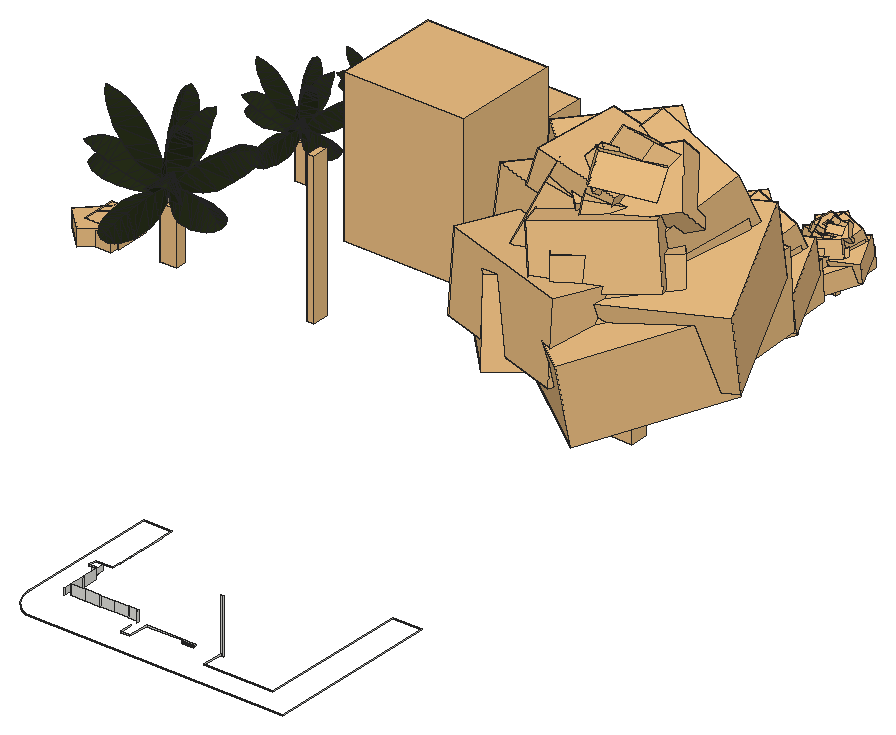
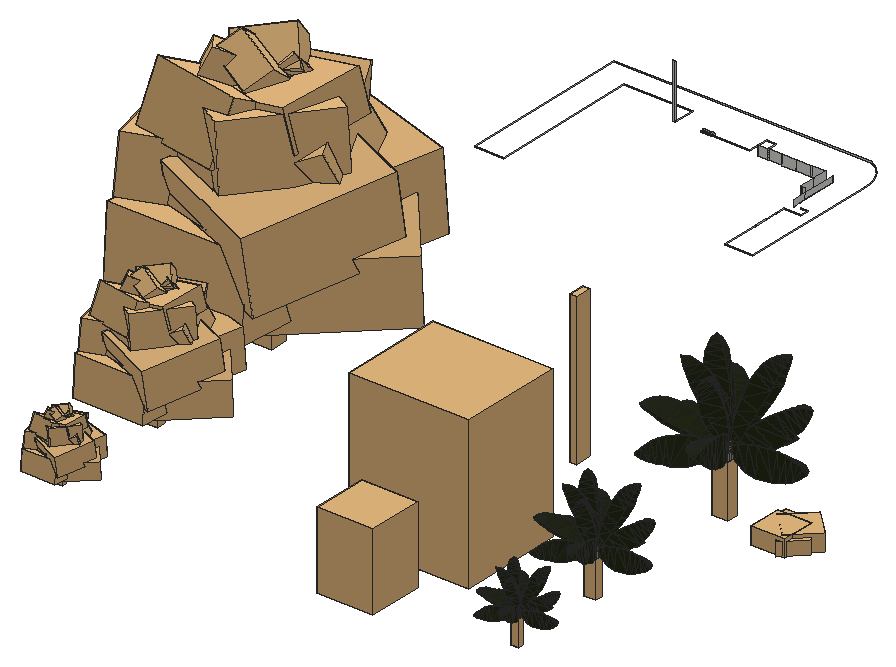
# SketchUp Ruby script. Lengths in inches.
U = 1.inch
M = Sketchup.active_model
def pt(a) = Geom::Point3d.new(a.map { |v| v * U })
def face(e, loops, mat)
  f = e.add_face(loops[0].map { |a| pt(a) })
  loops[1..].each { |l| e.add_face(l.map { |a| pt(a) }).erase! }
  f.material = f.back_material = mat if mat
  f
end
# faces: each face lists its corners as indices into pts; further lists are holes
def faces(e, pts, list, mat = nil) = list.each { |f| face(e, (f[0].is_a?(Array) ? f : [f]).map { |l| l.map { |i| pts[i] } }, mat) }
# xy, xz, yz: faces in a plane at the given z, y or x. An outline is a flat list of corners, or four numbers for a rectangle; further outlines are holes
def ring(l) = l.size == 4 ? [[l[0], l[1]], [l[2], l[1]], [l[2], l[3]], [l[0], l[3]]] : l.each_slice(2).to_a
def flat(e, list, mat, &to3) = list.each { |f| face(e, (f[0].is_a?(Array) ? f : [f]).map { |l| ring(l).map { |u, v| to3.(u, v) } }, mat) }
def xy(e, z, list, mat = nil) = flat(e, list, mat) { |x, y| [x, y, z] }
def xz(e, y, list, mat = nil) = flat(e, list, mat) { |x, z| [x, y, z] }
def yz(e, x, list, mat = nil) = flat(e, list, mat) { |y, z| [x, y, z] }
def lines(e, pts, list) = list.each { |a, b| e.add_line(pt(pts[a]), pt(pts[b])) }
# prism: a flat outline (further loops are holes) pulled along v
def prism(e, loops, v, mat = nil)
  f = face(e, loops, mat); d = Geom::Vector3d.new(v.map { |x| x * U })
  f.pushpull(f.normal.samedirection?(d) ? d.length : -d.length)
end
def box(e, o, s, mat = nil) = prism(e, [[o, [o[0] + s[0], o[1], o[2]], [o[0] + s[0], o[1] + s[1], o[2]], [o[0], o[1] + s[1], o[2]]]], [0, 0, s[2]], mat)
def at(x, y, z, deg = 0) = Geom::Transformation.translation(pt([x, y, z])) * Geom::Transformation.rotation(ORIGIN, Z_AXIS, deg.degrees)
def axes(o, x, y, z) = Geom::Transformation.new([*x, 0, *y, 0, *z, 0, *pt(o).to_a, 1])
def part(name) = M.definitions.add(name)
# library, detail: a bought-in or finely detailed component or shape, given as its bounding box
def library(name, o, s) = part(name).tap { |d| box(d.entities, o, s) }
def detail(e, o, s) = box(e.add_group.entities, o, s)
def put(e, d, t, mat = nil) = e.add_instance(d, t).tap { |i| i.material = mat if mat }
def group(e, t, mat = nil) = e.add_group.tap { |g| g.transformation = t; g.material = mat if mat }.entities
root = M.entities
M.materials.add("cocoanut_mat").color = [137, 122, 109]
M.materials.add("cocoanut_scrub").color = [165, 152, 134]
M.materials.add("coconut_test3_clean").color = [38, 45, 24]
c1 = library("Small Tree",[-46.3125,-47.83,0],[89.1875,89.28,122.02])
c2 = part("coconut_half")
p = [[54.48,2.6,2.17],[90.24,0,0],[105.09,35.75,42.48],[115.87,5,0],[128.48,35.75,36.0625],[152.37,21,0],
  [152.37,35.75,27.13],[169.19,35.75,17.77],[57.93,35.75,46.59],[42.36,5.25,5.16],[79.93,35.75,46.59],[41.85,35.75,44.23],
  [28.04,8.5,7.49],[27.85,35.75,39.58],[16.59,14.5,9.63],[9.27,35.75,26.98],[6.26,23.5,11.78],[16.71,35.75,32.89],
  [0,35.75,14.25]]
faces(c2.entities,p,[[0,1,2],[1,3,4],[1,4,2],[3,5,6],[3,6,4],[5,7,6],[0,8,9],[0,10,8],
  [0,2,10],[9,11,12],[9,8,11],[12,13,14],[12,11,13],[14,15,16],[14,17,15],[14,13,17],
  [18,16,15]],"coconut_test3_clean")
c3 = part("Group\#4")
put(c3.entities,c2,at(0,0,0))
put(c3.entities,c2,axes([0,71.5,0],[1,0,0],[0,-1,0],[0,0,1]))
c4 = part("coconut3_top")
put(c4.entities,c3,axes([-176.42,-40.5625,245.57],[1,0,0],[0,0.96593,-0.25882],[0,0.25882,0.96593]))
g1 = group(c4.entities,at(-4.7,-151.6,178.32))
put(g1,c2,axes([0,0,0],[0.14944,0.9543,0.25882],[-0.87562,0.00613,0.48296],[0.4593,-0.2988,0.83652]))
put(g1,c2,axes([-62.61,0.4375,34.53],[0.14944,0.9543,0.25882],[0.87562,-0.00613,-0.48296],[0.4593,-0.2988,0.83652]))
put(c4.entities,c3,axes([171.02,-15.64,245.06],[-0.94665,0.32227,0],[-0.31128,-0.91439,-0.25882],[-0.08341,-0.24501,0.96593]))
put(c4.entities,c3,axes([41.29,183.8,264.73],[-0.39574,-0.90582,-0.15126],[0.91636,-0.40035,0],[-0.06056,-0.13861,0.98849]))
put(c4.entities,c3,axes([-77.19,156.92,280.49],[0.30009,-0.91813,-0.25882],[0.86338,0.14605,0.48296],[-0.40562,-0.36839,0.83652]))
put(c4.entities,c3,axes([-112.56,-104.35,340.4],[0.76036,0.41456,-0.5],[-0.63406,0.64068,-0.43301],[0.14083,0.64627,0.75]))
put(c4.entities,c3,axes([119.49,-113.07,311.83],[-0.54618,0.67208,-0.5],[-0.83762,-0.43208,0.3342],[0.00857,0.60135,0.79894]))
put(c4.entities,c3,axes([103.27,116.54,337.13],[-0.75167,-0.49748,-0.43301],[0.65951,-0.56129,-0.5],[0.0057,-0.66141,0.75]))
put(c4.entities,c3,axes([-111.91,-75.47,434.48],[0.55528,0.30275,-1.09544],[-0.10884,0.68367,0.13377],[0.95166,0.05419,0.49738]))
put(c4.entities,c3,axes([96.22,-37.8,421.8],[-0.43628,0.34579,-0.96422],[-0.35338,-0.74638,-0.10777],[-0.75439,0.29273,0.44631]))
put(c4.entities,c3,axes([-41.59,80.66,420.02],[0.06101,-0.43197,-0.99256],[0.722,0.18761,-0.03727],[0.23024,-0.81295,0.36796]))
put(c4.entities,c3,axes([62.57,69.42,421.8],[-0.49424,-0.25619,-0.96422],[0.53593,-0.62829,-0.10777],[-0.57624,-0.5681,0.44631]))
c5 = part("cocoanut_mat")
yz(c5.entities,2,[[0.45,5,4.17,5,4.55,7.22,0,7.22]],"cocoanut_mat")
p = [[1.5,0.95,2.55],[0,1.26,0],[1.5,4.17,2.55],[0,3.01,0.06],[2,0.45,5],[2,4.17,5],
  [1.5,4.82,10.82],[1.5,0,9.97],[2,4.55,7.22],[2,0,7.22],[1,0.99,11.1],[1,3.98,11.36]]
faces(c5.entities,p,[[0,1,2],[3,2,1],[4,0,2,5],[6,7,8],[9,8,7],[7,6,10],[11,10,6]],"cocoanut_mat")
c6 = part("Coconut Palm")
xy(c6.entities,112.14,[[122.28,106.09,125.08,107.25,126.24,110.05,125.08,112.85,122.28,114.01,119.48,112.85,118.32,110.05,119.48,107.25]])
detail(c6.entities,[118.32,101.24,0],[25.61,17.45,83.17])
put(c6.entities,c4,axes([125.26,110.5,-76.06],[0.71,0,0],[0,0.71,0],[0,0,0.71]))
g2 = group(c6.entities,at(117.6,103.69,82.125))
p = [[4.68,2.4,1.05],[4.68,2.4,30.02],[1.88,3.56,30.02],[1.88,3.56,1.05],[7.48,3.56,1.05],[7.48,3.56,30.02],
  [0.72,6.36,30.02],[0.72,6.36,1.05],[8.64,6.36,1.05],[8.64,6.36,30.02],[1.88,9.16,30.02],[1.88,9.16,1.05],
  [7.48,9.16,1.05],[7.48,9.16,30.02],[4.68,10.32,30.02],[4.68,10.32,1.05]]
faces(g2,p,[[0,1,2,3],[4,5,1,0],[2,6,7,3],[4,8,9,5],[6,10,11,7],[8,12,13,9],[11,10,14,15],[15,14,13,12]],"cocoanut_scrub")
put(g2,c5,axes([8.73,9,14.81],[0.95137,0.17914,0.2506],[-0.24236,0.93742,0.25],[-0.19013,-0.29858,0.93525]))
put(g2,c5,axes([1.89,13.92,14.26],[-0.95388,0.23795,0.18301],[-0.27087,-0.94506,-0.18301],[0.17341,-0.30035,1.29434]))
put(g2,c5,axes([3.98,0.08,4.09],[0.521,-0.82169,0.23104],[0.85353,0.50368,-0.13339],[-0.00676,0.2667,0.96376]))
put(g2,c5,axes([2.8,2.4,6.76],[-0.16755,-0.98247,0.08171],[0.984,-0.16156,0.07513],[-0.09879,0.15157,1.61993]))
put(g2,c5,axes([8.29,10.47,4.97],[0.02489,0.99575,0.08868],[-0.99708,0.03112,-0.06968],[-0.11254,-0.13523,1.55005]))
put(g2,c5,axes([10.54,2.88,6.76],[0.95137,0.17914,0.2506],[-0.115,0.96125,-0.25056],[-0.28577,0.20956,0.9351]))
c7 = library("trunk\#1",[0,0,0],[11.46,27.17,238.43])
c8 = library("Group\#97",[-22.47,-14.25,0],[191.27,167.9,240.05])
c9 = library("Pine branch",[-164.19,86.97,62.64],[148.2,83.79,137.08])
c10 = part("Gruppe\#2")
detail(c10.entities,[0.71,-7.7,0],[22.57,19.31,263.85])
c11 = part("Kiefer Pine")
put(c11.entities,c9,axes([141.72,46.52,161.66],[-0.02916,-0.63772,0.00271],[0.15221,-0.00358,0.48358],[-0.6193,0.02915,0.11872]))
put(c11.entities,c9,axes([97.98,30.67,99.84],[-0.47537,-0.59297,0.00413],[0.14389,-0.11021,0.73807],[-0.57526,0.46243,0.1812]))
put(c11.entities,c9,axes([147.43,170.77,85.84],[0.66331,0.36209,0.08066],[-0.16152,0.13314,0.73061],[0.33395,-0.6548,0.19316]))
put(c11.entities,c9,axes([126.12,172.51,50.8],[0.58404,0.48629,0.00413],[-0.11903,0.13668,0.73807],[0.47151,-0.56784,0.1812]))
put(c11.entities,c9,axes([129.28,102.66,199.18],[0.3329,0.20176,-0.07756],[-0.04952,0.23763,0.27741],[0.2165,-0.24552,0.14305]))
put(c11.entities,c9,axes([28.39,91.46,58.6],[-0.71464,0.25212,0.05767],[-0.01186,-0.20123,0.73278],[0.25836,0.68814,0.19316]))
put(c11.entities,c9,axes([152.74,49.28,68.93],[0.33164,-0.67512,0.10878],[0.24998,0.23222,0.67911],[-0.63649,-0.26056,0.32339]))
put(c11.entities,c9,axes([-6.13,166.4,41.09],[-0.38774,0.8952,0.21972],[0.05521,-0.21538,0.97497],[0.92011,0.39016,0.03409]))
put(c11.entities,c9,axes([103.12,114.79,195.58],[-0.35402,0.16187,-0.07756],[-0.18541,-0.24864,0.1992],[0.04135,0.27092,0.22915]))
put(c11.entities,c9,axes([201.4375,150.2,7.87],[0.95266,-0.30403,0],[0.02078,0.06511,0.99766],[-0.30332,-0.95043,0.06835]))
put(c11.entities,c9,axes([149.14,-15.51,56.65],[-0.38076,-0.9108,0.15959],[0.00531,0.17044,0.98535],[-0.92466,0.37603,-0.06006]))
put(c11.entities,c9,axes([123.6,85.97,205.1],[0.23507,-0.19426,-0.06076],[0.16806,0.10538,0.1906],[-0.12474,-0.2241,0.1423]))
put(c11.entities,c9,axes([121.72,132.51,172.5],[0.36293,0.20783,-0.0399],[0.00027,0.10027,0.31921],[0.21403,-0.35254,0.06727]))
put(c11.entities,c9,axes([57.2,144.19,196.7],[-0.28797,0.37098,0.1914],[-0.03125,-0.30847,0.33516],[0.44369,0.21905,0.14782]))
put(c11.entities,c9,axes([93.55,232.34,18.61],[0.58552,0.78879,0.18704],[-0.06218,-0.18635,0.98051],[0.80827,-0.58574,-0.06006]))
put(c11.entities,c9,axes([33.34,105.32,91.71],[-0.72171,0.22385,0.08143],[-0.02606,-0.33247,0.68293],[0.23677,0.64572,0.32339]))
put(c11.entities,c9,axes([227.44,74.67,9.76],[0.6363,-0.72678,0.25867],[-0.14373,0.21775,0.96536],[-0.75793,-0.65144,0.03409]))
put(c11.entities,c9,axes([24.14,28.375,-27.51],[-1,0,0],[0,-0.06835,0.99766],[0,0.99766,0.06835]))
put(c11.entities,c10,at(97.66,98.27,0))
c12 = library("Grass - Sedge  3D",[-3.65,-3.5625,-0.25],[6.94,6.99,3.41])
xy(root,0,[[564.74,183.7,565.04,248.89],[565.04,237.58,565.41,237.58,565.41,241.02,565.16,241.02,565.16,261.08,565.04,261.08],[564.49,248.89,565.04,261.08]])
xz(root,113.86,[[560.04,0,967.75,1.5625]])
xz(root,152.69,[[679.09,0,694.73,1.5625],[812.47,0,921.28,1.5625]])
xz(root,179.27,[[755.09,0,756.79,1.5625],[757.59,0,759.29,1.5625],[760.09,0,761.79,1.5625],[762.59,0,764.29,1.5625],[765.09,0,766.79,1.5625],
  [767.59,0,769.29,1.5625],[770.09,0,771.79,1.5625],[772.59,0,774.29,1.5625]])
xz(root,184.77,[[694.73,0,755.09,1.5625],[756.79,0,757.59,1.5625],[759.29,0,760.09,1.5625],[761.79,0,762.59,1.5625],[764.29,0,765.09,1.5625],
  [766.79,0,767.59,1.5625],[769.29,0,770.09,1.5625],[771.79,0,772.59,1.5625],[812.72,0,814.41,86.125],[815.59,0,817.29,86.125]])
xz(root,188.52,[[572.41,0,593.95,16.125],[593.95,0,594.71,16.125],[594.71,0,618.47,16.125],[618.47,0,619.6,16.125],[619.6,0,641.13,16.125],
  [641.13,0,642.0625,16.125],[642.0625,0,662.45,16.125],[662.45,0,663.59,16.125],[663.59,0,679.09,16.125]])
xz(root,237.58,[[565.41,0,570.41,16.125],[570.41,0,572.41,16.125]])
xz(root,261.08,[[542.91,0,553.86,1.5625]])
xz(root,273.58,[[542.91,0,570.41,1.5625]])
xz(root,390.8,[[525.25,0,570.41,1.5625],[921.28,0,967.75,1.5625]])
yz(root,525.25,[[162.48,0,171.1,1.5625],[171.1,0,390.8,1.5625]])
yz(root,542.91,[[261.08,0,273.58,1.5625]])
yz(root,565.04,[[183.7,0,184.6,9.25],[184.6,0,237.58,9.25],[237.58,0,261.08,9.25]])
yz(root,570.41,[[273.58,0,288.11,1.5625],[288.11,0,288.9,1.5625],[288.9,0,307.55,1.5625],[307.55,0,308.36,1.5625],[308.36,0,329.67,1.5625],
  [329.67,0,330.36,1.5625],[330.36,0,350.49,1.5625],[350.49,0,350.93,1.5625],[350.93,0,370.6875,1.5625],[370.6875,0,371.49,1.5625],
  [371.49,0,390.8,1.5625]])
yz(root,572.41,[[188.52,0,211.54,16.125],[211.54,0,213.05,16.125],[213.05,0,237.58,16.125]])
yz(root,679.09,[[152.69,0,173.38,1.5625],[184.6,0,184.77,16.125],[184.77,0,188.52,16.125]])
yz(root,694.73,[[152.69,0,184.77,1.5625]])
yz(root,755.09,[[179.27,0,184.77,1.5625]])
yz(root,756.79,[[179.27,0,184.77,1.5625]])
yz(root,757.59,[[179.27,0,184.77,1.5625]])
yz(root,759.29,[[179.27,0,184.77,1.5625]])
yz(root,760.09,[[179.27,0,184.77,1.5625]])
yz(root,761.79,[[179.27,0,184.77,1.5625]])
yz(root,762.59,[[179.27,0,184.77,1.5625]])
yz(root,764.29,[[179.27,0,184.77,1.5625]])
yz(root,765.09,[[179.27,0,184.77,1.5625]])
yz(root,766.79,[[179.27,0,184.77,1.5625]])
yz(root,767.59,[[179.27,0,184.77,1.5625]])
yz(root,769.29,[[179.27,0,184.77,1.5625]])
yz(root,770.09,[[179.27,0,184.77,1.5625]])
yz(root,771.79,[[179.27,0,184.77,1.5625]])
yz(root,772.59,[[179.27,0,184.77,1.5625]])
yz(root,812.47,[[152.69,0,184.77,1.5625]])
yz(root,921.28,[[152.69,0,390.8,1.5625]])
yz(root,967.75,[[113.86,0,390.8,1.5625]])
p = [[554.66,116.43,0],[560.04,113.86,0],[560.04,113.86,1.5625],[554.66,116.43,1.5625],[549.57,119.56,0],[549.57,119.56,1.5625],
  [544.85,123.2,0],[544.85,123.2,1.5625],[540.53,127.32,0],[540.53,127.32,1.5625],[536.66,131.87,0],[536.66,131.87,1.5625],
  [533.3,136.8,0],[533.3,136.8,1.5625],[530.47,142.06,0],[530.47,142.06,1.5625],[528.21,147.58,0],[528.21,147.58,1.5625],
  [526.54,153.3125,0],[526.54,153.3125,1.5625],[525.49,159.18,0],[525.49,159.18,1.5625],[525.25,162.48,0],[525.25,162.48,1.5625]]
faces(root,p,[[0,1,2,3],[4,0,3,5],[6,4,5,7],[8,6,7,9],[10,8,9,11],[12,10,11,13],[14,12,13,15],[16,14,15,17],
  [18,16,17,19],[20,18,19,21],[22,20,21,23]])
put(root,c1,at(372.57,1353.29,0))
put(root,c6,at(12.56,816,0))
put(root,c6,axes([51.13,1110.27,0],[0.7,0,0],[0,0.7,0],[0,0,0.7]))
put(root,c6,axes([76.23,1288.91,0],[0.483,0,0],[0,0.483,0],[0,0,0.483]))
put(root,c7,at(367,912.29,0))
put(root,c8,at(297.47,1115.07,0))
put(root,c11,axes([794.84,1338.75,0],[0.375,0,0],[0,0.375,0],[0,0,0.375]))
put(root,c11,axes([758.14,1109.03,0],[0.75,0,0],[0,0.75,0],[0,0,0.75]))
put(root,c11,axes([696.28,784.68,0],[1.5,0,0],[0,1.5,0],[0,0,1.5]))
put(root,c12,axes([44.57,937.38,1.92],[0,7.7292,0],[-7.7292,0,0],[0,0,7.7292]))
put(root,c12,axes([27.72,920.13,1.92],[5.46537,5.46537,0],[-5.46537,5.46537,0],[0,0,7.7292]))
put(root,c12,axes([26.39,937.79,1.58],[-4.49805,4.49805,0],[-4.49805,-4.49805,0],[0,0,6.3612]))
put(root,c12,axes([44.35,921.36,1.7],[0,6.84,0],[-6.84,0,0],[0,0,6.84]))
